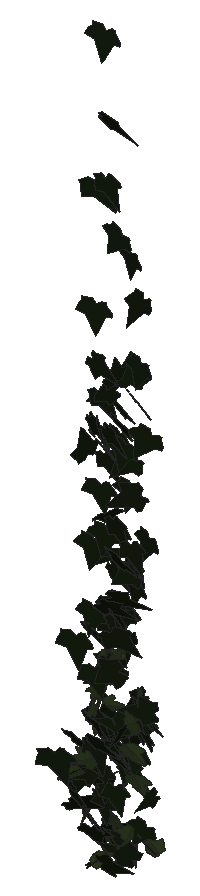
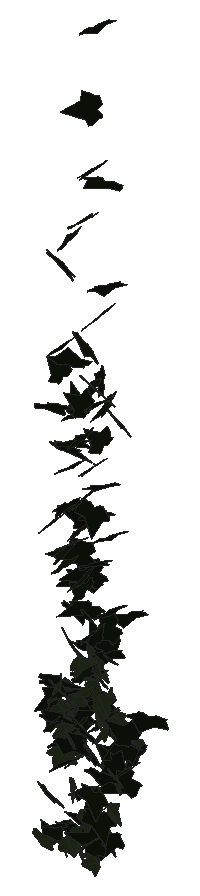
# SketchUp Ruby script. Lengths in inches.
U = 1.inch
M = Sketchup.active_model
def pt(a) = Geom::Point3d.new(a.map { |v| v * U })
def face(e, loops, mat)
  f = e.add_face(loops[0].map { |a| pt(a) })
  loops[1..].each { |l| e.add_face(l.map { |a| pt(a) }).erase! }
  f.material = f.back_material = mat if mat
  f
end
# faces: each face lists its corners as indices into pts; further lists are holes
def faces(e, pts, list, mat = nil) = list.each { |f| face(e, (f[0].is_a?(Array) ? f : [f]).map { |l| l.map { |i| pts[i] } }, mat) }
# xy, xz, yz: faces in a plane at the given z, y or x. An outline is a flat list of corners, or four numbers for a rectangle; further outlines are holes
def ring(l) = l.size == 4 ? [[l[0], l[1]], [l[2], l[1]], [l[2], l[3]], [l[0], l[3]]] : l.each_slice(2).to_a
def flat(e, list, mat, &to3) = list.each { |f| face(e, (f[0].is_a?(Array) ? f : [f]).map { |l| ring(l).map { |u, v| to3.(u, v) } }, mat) }
def xy(e, z, list, mat = nil) = flat(e, list, mat) { |x, y| [x, y, z] }
def xz(e, y, list, mat = nil) = flat(e, list, mat) { |x, z| [x, y, z] }
def yz(e, x, list, mat = nil) = flat(e, list, mat) { |y, z| [x, y, z] }
def lines(e, pts, list) = list.each { |a, b| e.add_line(pt(pts[a]), pt(pts[b])) }
# prism: a flat outline (further loops are holes) pulled along v
def prism(e, loops, v, mat = nil)
  f = face(e, loops, mat); d = Geom::Vector3d.new(v.map { |x| x * U })
  f.pushpull(f.normal.samedirection?(d) ? d.length : -d.length)
end
def box(e, o, s, mat = nil) = prism(e, [[o, [o[0] + s[0], o[1], o[2]], [o[0] + s[0], o[1] + s[1], o[2]], [o[0], o[1] + s[1], o[2]]]], [0, 0, s[2]], mat)
def at(x, y, z, deg = 0) = Geom::Transformation.translation(pt([x, y, z])) * Geom::Transformation.rotation(ORIGIN, Z_AXIS, deg.degrees)
def axes(o, x, y, z) = Geom::Transformation.new([*x, 0, *y, 0, *z, 0, *pt(o).to_a, 1])
def part(name) = M.definitions.add(name)
# library, detail: a bought-in or finely detailed component or shape, given as its bounding box
def library(name, o, s) = part(name).tap { |d| box(d.entities, o, s) }
def detail(e, o, s) = box(e.add_group.entities, o, s)
def put(e, d, t, mat = nil) = e.add_instance(d, t).tap { |i| i.material = mat if mat }
def group(e, t, mat = nil) = e.add_group.tap { |g| g.transformation = t; g.material = mat if mat }.entities
root = M.entities
M.materials.add("1026 AP 7946 SUNNY SIDE UP").color = [254, 231, 186]
M.materials.add("efeu1").color = [18, 25, 13]
M.materials.add("efeu2").color = [43, 57, 29]
c1 = part("ivyleaf_9")
p = [[1.54,2.16,1.25],[1.36,2.04,1.19],[-0.21,0.99,0.68],[-0.71,1.11,0.82],[-0.85,0.86,0.67],[-0.8,0.17,0.21],
  [-0.9,-0.01,0.1],[-0.67,-0.16,-0.02],[-0.08,-0.08,-0.05],[-0.03,-0.6,-0.4],[0.65,-0.88,-0.66],[0.83,-0.6,-0.49],
  [1.29,-0.42,-0.43],[1.8125,-0.07,-0.26],[1.21,0.44,0.15]]
faces(c1.entities,p,[[0,1,2,3,4,5,6,7,8,9,10,11,12,13,14]],"efeu1")
c2 = part("ivyleaf_10")
p = [[0,0.5,-0.03],[-0.0625,2.02,-0.43],[-0.19,2.01,-0.46],[-0.54,1.05,-0.29],[-0.52,0.625,-0.18],[-0.83,0.76,-0.28],
  [-1.16,0.64,-0.33],[-1.15,0.33,-0.24],[-0.77,-0.39,0.02],[-0.3,-0.51,0.16],[0.04,-0.48,0.23],[-0.02,2.01,-0.4375],
  [-0.06,2.01,-0.43],[0.04,-0.49,0.23],[0.67,-0.49,0.14],[1.38,0.36,-0.2],[1.375,0.51,-0.24],[0.81,0.65,-0.19],
  [0.62,0.59,-0.15],[0.6,1.09,-0.28],[0.5,1.23,-0.31]]
faces(c2.entities,p,[[0,1,2,3,4,5,6,7,8,9,10],[11,12,0,13,14,15,16,17,18,19,20]],"efeu2")
put(root,c1,axes([145.4,211.73,293.24],[0.1308,0.39329,-0.08465],[-0.1128,-0.0703,-0.41072],[-0.62235,0.0954,0.05665]),"1026 AP 7946 SUNNY SIDE UP")
put(root,c1,axes([145.09,212.38,332.73],[-0.18968,-0.4622,0.05841],[-0.00333,-0.06074,-0.49227],[0.73272,-0.11993,0.01288]),"1026 AP 7946 SUNNY SIDE UP")
put(root,c1,axes([145.11,210.46,294.86],[-0.13222,-0.37976,0.22466],[-0.00281,-0.22394,-0.39982],[0.69028,-0.07365,0.04141]),"1026 AP 7946 SUNNY SIDE UP")
put(root,c1,axes([144.88,211.98,324.96],[-0.12009,-0.34192,-0.3066],[0.40064,0.21513,-0.32283],[0.58711,-0.21674,0.15758]),"1026 AP 7946 SUNNY SIDE UP")
put(root,c2,axes([145.25,211.95,298.35],[0.15557,-0.32161,0.2261],[0.14455,-0.20269,-0.34697],[0.59659,0.13298,0.02511]),"1026 AP 7946 SUNNY SIDE UP")
put(root,c2,axes([145.39,211.61,298.87],[-0.15556,-0.36875,0.11832],[0.00302,-0.12118,-0.39266],[0.60828,-0.0937,0.03221]),"1026 AP 7946 SUNNY SIDE UP")
put(root,c1,axes([145.07,212.01,313.98],[0.16538,-0.40483,-0.15305],[0.02148,0.15363,-0.42704],[0.67649,0.09409,0.05097]),"1026 AP 7946 SUNNY SIDE UP")
put(root,c1,axes([144.89,210.25,296.61],[0.18386,-0.18869,0.33919],[0.40692,-0.21384,-0.22146],[0.43844,0.2776,0.0633]),"1026 AP 7946 SUNNY SIDE UP")
put(root,c2,axes([145.41,210.74,294.76],[0.45615,-0.26317,-0.04835],[-0.06624,0.02115,-0.40318],[0.41467,0.29287,-0.01122]),"1026 AP 7946 SUNNY SIDE UP")
put(root,c1,axes([145.48,212.25,305.9],[-0.40948,-0.27532,0.17153],[-0.06851,-0.184,-0.38115],[0.50255,-0.24941,0.08781]),"1026 AP 7946 SUNNY SIDE UP")
put(root,c1,axes([145.36,211.19,303.09],[-0.1702,-0.41187,0.10357],[-0.02747,-0.10175,-0.43922],[0.66695,-0.1093,0.00834]),"1026 AP 7946 SUNNY SIDE UP")
put(root,c1,axes([145.66,211.73,294.24],[0.0959,0.40449,0.06801],[-0.05457,0.0693,-0.41855],[-0.64155,0.05457,0.04577]),"1026 AP 7946 SUNNY SIDE UP")
put(root,c1,axes([145.59,211.95,300.43],[-0.51018,0.06694,-0.20722],[0.27988,-0.11498,-0.33523],[-0.1821,-0.36424,0.06532]),"1026 AP 7946 SUNNY SIDE UP")
put(root,c2,axes([145.53,210.68,292.96],[0.1252,-0.3432,0.1834],[0.03262,-0.1797,-0.36352],[0.60848,0.08025,-0.01825]),"1026 AP 7946 SUNNY SIDE UP")
put(root,c1,axes([145.24,212.11,302.15],[0.01326,-0.15045,0.38291],[0.13284,-0.36363,-0.15538],[0.61764,0.08144,0.0252]),"1026 AP 7946 SUNNY SIDE UP")
put(root,c1,axes([145.28,208.47,296.72],[-0.28793,-0.29848,-0.31991],[0.28394,0.25112,-0.35886],[0.61277,-0.25661,0.01597]),"1026 AP 7946 SUNNY SIDE UP")
put(root,c2,axes([145.47,211.23,297.21],[0.07716,-0.18653,-0.33902],[0.17216,0.32359,-0.1708],[0.56782,-0.07277,0.09785]),"1026 AP 7946 SUNNY SIDE UP")
put(root,c1,axes([145.94,209.99,312.04],[-0.55606,0.1642,-0.2813],[-0.36796,0.14504,0.40155],[0.34186,0.42319,-0.02534]),"1026 AP 7946 SUNNY SIDE UP")
put(root,c1,axes([145.52,210.85,291.88],[0.53458,0.1874,-0.12745],[-0.14661,-0.08851,-0.39917],[-0.32223,0.35117,-0.02983]),"1026 AP 7946 SUNNY SIDE UP")
put(root,c1,axes([145.43,209.77,302.31],[-0.19687,-0.44602,-0.09483],[0.06061,0.08211,-0.47653],[0.71274,-0.13018,0.01433]),"1026 AP 7946 SUNNY SIDE UP")
put(root,c1,axes([145.23,210.91,302.28],[0.6684,-0.16731,0.0066],[-0.01286,-0.04079,-0.46896],[0.26302,0.42318,-0.03971]),"1026 AP 7946 SUNNY SIDE UP")
put(root,c1,axes([145.48,211.08,306.72],[-0.22883,-0.42799,0.09691],[0.04251,-0.11023,-0.46226],[0.68855,-0.13543,0.06075]),"1026 AP 7946 SUNNY SIDE UP")
put(root,c1,axes([145.33,212.07,310.74],[0.2031,-0.39692,-0.07272],[0.00769,0.07331,-0.42868],[0.63325,0.12641,0.02853]),"1026 AP 7946 SUNNY SIDE UP")
put(root,c1,axes([145.26,209.25,295.16],[0.28788,-0.38308,0.20038],[0.115,-0.18295,-0.4383],[0.66727,0.1968,-0.01091]),"1026 AP 7946 SUNNY SIDE UP")
put(root,c1,axes([145.375,211.17,297.76],[0.30067,-0.38391,-0.08821],[-0.03819,0.08108,-0.44113],[0.61657,0.19224,0.01569]),"1026 AP 7946 SUNNY SIDE UP")
put(root,c1,axes([145.77,212.08,300],[-0.42041,-0.21348,0.20522],[-0.06404,-0.24165,-0.32255],[0.45595,-0.23078,0.14392]),"1026 AP 7946 SUNNY SIDE UP")
put(root,c1,axes([145.63,212.07,296.44],[-0.42852,0.00274,-0.2749],[0.41272,-0.06625,-0.27722],[-0.07591,-0.37563,0.04462]),"1026 AP 7946 SUNNY SIDE UP")
put(root,c1,axes([145.47,211.54,309.49],[-0.17974,-0.40186,-0.05058],[0.16311,0.01791,-0.41921],[0.6149,-0.12222,0.09642]),"1026 AP 7946 SUNNY SIDE UP")
put(root,c2,axes([145.43,212.05,291.04],[-0.32019,0.13339,-0.28193],[0.32063,-0.18594,-0.25008],[-0.35692,-0.28671,0.02827]),"1026 AP 7946 SUNNY SIDE UP")
put(root,c2,axes([146.01,209.11,295.79],[-0.268,-0.16531,0.31513],[-0.31549,-0.23274,-0.24536],[0.44811,-0.26273,0.01572]),"1026 AP 7946 SUNNY SIDE UP")
put(root,c1,axes([145.5625,211.1,319.15],[-0.2273,-0.4294,-0.04684],[0.0609,0.03228,-0.46578],[0.67583,-0.14732,0.02622]),"1026 AP 7946 SUNNY SIDE UP")
put(root,c1,axes([145.28,211.66,311.65],[0.18043,-0.28624,0.32071],[0.25963,-0.26845,-0.31691],[0.61424,0.19755,0.03975]),"1026 AP 7946 SUNNY SIDE UP")
put(root,c1,axes([146.11,211.74,314.55],[-0.59694,0.20463,0.01218],[-0.04521,-0.03096,-0.44247],[-0.31901,-0.37852,0.0399]),"1026 AP 7946 SUNNY SIDE UP")
put(root,c2,axes([145.68,210.69,298.47],[-0.01509,0.18356,-0.36487],[-0.01803,-0.35531,-0.19091],[-0.62846,0.00579,0.01424]),"1026 AP 7946 SUNNY SIDE UP")
put(root,c1,axes([145.52,211.89,302.38],[0.17239,-0.39335,-0.11439],[-0.05308,0.10354,-0.42004],[0.63953,0.11462,-0.00402]),"1026 AP 7946 SUNNY SIDE UP")
put(root,c2,axes([145.81,211.88,301.28],[0.189,-0.37946,-0.0446],[-0.01724,0.03968,-0.40983],[0.59992,0.12068,0.00227]),"1026 AP 7946 SUNNY SIDE UP")
put(root,c1,axes([145.53,210.83,313.25],[0.43819,-0.3393,-0.1565],[-0.18412,0.09756,-0.4509],[0.5535,0.30107,-0.02609]),"1026 AP 7946 SUNNY SIDE UP")
put(root,c1,axes([145.87,211.48,308.18],[0.18559,0.40275,-0.01505],[0.0127,-0.01997,-0.43225],[-0.63371,0.11755,-0.01307]),"1026 AP 7946 SUNNY SIDE UP")
put(root,c2,axes([146.17,210.93,300.2],[-0.30728,0.12904,0.33727],[-0.50995,0.0772,-0.23084],[-0.21199,-0.37274,0.06642]),"1026 AP 7946 SUNNY SIDE UP")
put(root,c1,axes([145.53,211.9,325.35],[0.13081,-0.44557,-0.0839],[0.00104,0.08035,-0.46622],[0.71151,0.0818,0.01611]),"1026 AP 7946 SUNNY SIDE UP")
put(root,c1,axes([145.66,211.54,293.1875],[-0.01039,-0.4155,0.06784],[0.00443,-0.06826,-0.42849],[0.66207,-0.00606,0.00393]),"1026 AP 7946 SUNNY SIDE UP")
put(root,c1,axes([145.68,209.13,295.44],[0.38112,0.25895,0.32085],[0.28705,0.25225,-0.36266],[-0.56654,0.302,0.03209]),"1026 AP 7946 SUNNY SIDE UP")
put(root,c1,axes([145.81,211.14,294.9375],[-0.43462,-0.18419,-0.20121],[0.29365,0.06741,-0.33917],[0.3016,-0.33105,0.04027]),"1026 AP 7946 SUNNY SIDE UP")
put(root,c1,axes([145.6,209.36,293.93],[0.50397,0.25496,0.25675],[0.31491,0.14616,-0.42097],[-0.4619,0.37783,-0.00687]),"1026 AP 7946 SUNNY SIDE UP")
put(root,c1,axes([145.37,212.04,328.4],[0.64545,-0.17249,0.17587],[0.22296,-0.10411,-0.45761],[0.31102,0.4326,-0.03693]),"1026 AP 7946 SUNNY SIDE UP")
put(root,c2,axes([145.77,211.98,300.59],[-0.53482,-0.1193,-0.14946],[0.27223,-0.086,-0.34742],[0.1124,-0.35936,0.1303]),"1026 AP 7946 SUNNY SIDE UP")
put(root,c1,axes([145.52,210.43,294.95],[0.0775,-0.14359,0.43338],[0.34457,-0.36134,-0.15532],[0.6095,0.22253,0.0327]),"1026 AP 7946 SUNNY SIDE UP")
put(root,c1,axes([145.68,212.38,300.34],[-0.00973,-0.28146,0.28772],[0.18315,-0.26988,-0.27753],[0.59782,0.0781,0.08971]),"1026 AP 7946 SUNNY SIDE UP")
put(root,c1,axes([146.25,210.93,291.22],[0.02533,0.02127,-0.37175],[-0.5288,0.13366,-0.00657],[0.20893,0.3357,0.02845]),"1026 AP 7946 SUNNY SIDE UP")
put(root,c1,axes([145.99,211.38,294.03],[0.18726,-0.1966,-0.37698],[-0.37293,0.27893,-0.23299],[0.53435,0.26357,-0.0305]),"1026 AP 7946 SUNNY SIDE UP")
put(root,c1,axes([145.71,211.33,291.61],[0.18689,0.33229,-0.2399],[0.05319,0.23565,0.36265],[0.63751,-0.11707,0.04007]),"1026 AP 7946 SUNNY SIDE UP")
put(root,c1,axes([145.8,212.04,305.14],[0.37061,-0.30754,-0.16514],[-0.12408,0.13901,-0.39781],[0.52973,0.24772,0.02236]),"1026 AP 7946 SUNNY SIDE UP")
put(root,c1,axes([145.93,211.78,291.68],[0.05895,-0.39281,0.03123],[-0.0112,-0.03337,-0.40657],[0.61968,0.03677,-0.01032]),"1026 AP 7946 SUNNY SIDE UP")
put(root,c1,axes([145.78,211.9,303.54],[0.10656,-0.18606,-0.4052],[0.2259,0.38426,-0.15995],[0.64421,-0.10397,0.12311]),"1026 AP 7946 SUNNY SIDE UP")
put(root,c1,axes([146.11,211.75,300.13],[-0.23541,-0.22303,0.30846],[-0.02951,-0.31896,-0.25522],[0.58792,-0.10531,0.1107]),"1026 AP 7946 SUNNY SIDE UP")
put(root,c1,axes([145.92,212.37,311.92],[0.02126,-0.38333,0.20397],[0.05638,-0.19858,-0.39544],[0.67764,0.02855,0.0265]),"1026 AP 7946 SUNNY SIDE UP")
put(root,c1,axes([146,210.45,300.48],[-0.15253,-0.37922,-0.17789],[0.08303,0.16245,-0.40217],[0.64851,-0.11,0.00965]),"1026 AP 7946 SUNNY SIDE UP")
put(root,c1,axes([146.34,211.43,299.73],[-0.52024,-0.15728,0.2068],[0.2547,0.12624,0.37599],[-0.31114,0.36631,-0.03799]),"1026 AP 7946 SUNNY SIDE UP")
put(root,c1,axes([146.6,209.41,295.91],[-0.63242,0.05212,0.11565],[-0.18362,-0.03636,-0.41493],[-0.06319,-0.41591,0.04828]),"1026 AP 7946 SUNNY SIDE UP")
put(root,c2,axes([146.18,212.1,300.73],[-0.17412,-0.36506,-0.07141],[0.11549,0.04724,-0.38851],[0.57213,-0.12064,0.05669]),"1026 AP 7946 SUNNY SIDE UP")
put(root,c1,axes([145.96,211.92,291.69],[0.0322,-0.40453,-0.0049],[0.06453,0.00452,-0.41508],[0.63281,0.02012,0.04258]),"1026 AP 7946 SUNNY SIDE UP")
put(root,c1,axes([146.16,212.18,322.52],[-0.27644,-0.31495,0.29124],[-0.0408,-0.29938,-0.35971],[0.66611,-0.14904,0.09883]),"1026 AP 7946 SUNNY SIDE UP")
put(root,c1,axes([145.75,212.26,313.55],[0.25219,-0.24995,0.33855],[0.2689,-0.28235,-0.30755],[0.59287,0.23438,-0.00452]),"1026 AP 7946 SUNNY SIDE UP")
put(root,c2,axes([146.64,209.22,296.63],[-0.34999,-0.00463,0.33],[-0.47793,-0.12028,-0.22006],[0.15929,-0.37108,0.06481]),"1026 AP 7946 SUNNY SIDE UP")
put(root,c1,axes([146.22,211.08,307.57],[-0.30368,-0.37008,-0.009],[0.03388,-0.00377,-0.42953],[0.58102,-0.19321,0.02034]),"1026 AP 7946 SUNNY SIDE UP")
put(root,c1,axes([146.1,212.125,307.28],[0.07597,-0.40901,0.12389],[0.01978,-0.12194,-0.425],[0.6711,0.04989,-0.0015]),"1026 AP 7946 SUNNY SIDE UP")
put(root,c2,axes([146.53,211.22,292.64],[-0.48675,0.19775,0.09001],[-0.15265,0.00703,-0.37551],[-0.30294,-0.32127,0.0446]),"1026 AP 7946 SUNNY SIDE UP")
put(root,c1,axes([146.36,211.53,296.86],[-0.42125,0.2828,0.18151],[0.21295,-0.11188,0.40015],[0.47722,0.29955,-0.01834]),"1026 AP 7946 SUNNY SIDE UP")
put(root,c1,axes([146.83,212.1,296.7],[-0.07035,0.12268,-0.37154],[-0.29523,-0.32382,-0.0912],[-0.52239,0.16648,0.10158]),"1026 AP 7946 SUNNY SIDE UP")
put(root,c1,axes([146.86,210.95,315.82],[-0.48085,0.17834,-0.32537],[-0.38099,0.20873,0.36317],[0.42626,0.38774,-0.04245]),"1026 AP 7946 SUNNY SIDE UP")
put(root,c1,axes([146.81,209.69,291.19],[-0.17304,0.36837,0.00013],[-0.02155,-0.00615,-0.39581],[-0.57884,-0.10989,0.0147]),"1026 AP 7946 SUNNY SIDE UP")
put(root,c1,axes([146.43,211.375,294.01],[-0.09709,-0.37121,-0.12306],[0.06119,0.11233,-0.38651],[0.60909,-0.07046,0.01921]),"1026 AP 7946 SUNNY SIDE UP")
put(root,c1,axes([146.58,211.02,298.4],[-0.19186,-0.09951,0.44541],[-0.13185,-0.43573,-0.13007],[0.68592,-0.11159,0.09959]),"1026 AP 7946 SUNNY SIDE UP")
put(root,c1,axes([146.97,211.23,300.57],[-0.52339,0.20405,-0.00247],[-0.02187,-0.02946,-0.401],[-0.32014,-0.33157,0.03142]),"1026 AP 7946 SUNNY SIDE UP")
put(root,c1,axes([146.25,208.75,294.81],[0.32621,-0.37272,0.15984],[0.09945,-0.14469,-0.44005],[0.62828,0.21642,-0.01334]),"1026 AP 7946 SUNNY SIDE UP")
put(root,c2,axes([146.72,211.94,294.49],[0.15685,-0.31105,-0.20951],[-0.04294,0.20204,-0.33387],[0.58125,0.09886,0.03187]),"1026 AP 7946 SUNNY SIDE UP")
put(root,c1,axes([146.68,211.87,303.16],[-0.54754,-0.07765,-0.19756],[0.30397,0.00923,-0.36626],[0.11411,-0.39721,0.0277]),"1026 AP 7946 SUNNY SIDE UP")
put(root,c2,axes([146.49,210.67,298.75],[-0.09864,-0.10888,-0.39494],[0.34494,0.31381,-0.12717],[0.52203,-0.22793,0.0094]),"1026 AP 7946 SUNNY SIDE UP")
put(root,c1,axes([146.42,209.91,317.1],[0.40131,-0.28761,-0.26896],[-0.14506,0.25662,-0.38506],[0.59152,0.25806,0.08804]),"1026 AP 7946 SUNNY SIDE UP")
put(root,c2,axes([146.81,212.1,291.64],[-0.30666,-0.28547,0.13304],[-0.01588,-0.14815,-0.34958],[0.49347,-0.18217,0.07143]),"1026 AP 7946 SUNNY SIDE UP")
put(root,c1,axes([147.14,210.72,300.66],[-0.71468,0.00813,0.1115],[-0.17055,-0.04525,-0.46618],[0.0041,-0.46502,0.04456]),"1026 AP 7946 SUNNY SIDE UP")
put(root,c1,axes([146.51,209.89,297.02],[0.02895,-0.45955,-0.06584],[-0.02807,0.0606,-0.47319],[0.72845,0.0206,-0.01562]),"1026 AP 7946 SUNNY SIDE UP")
put(root,c2,axes([146.69,212.23,296.96],[0.40403,-0.26976,0.08557],[0.06355,-0.07809,-0.38346],[0.43997,0.259,-0.02319]),"1026 AP 7946 SUNNY SIDE UP")
put(root,c2,axes([146.53,210.08,291.01],[0.24999,0.21737,0.28113],[0.2005,0.24148,-0.27453],[-0.509,0.20188,0.02993]),"1026 AP 7946 SUNNY SIDE UP")
put(root,c1,axes([146.57,212.39,321.59],[0.01868,-0.38663,0.25678],[-0.00681,-0.25161,-0.39982],[0.72516,0.0076,-0.01037]),"1026 AP 7946 SUNNY SIDE UP")
put(root,c2,axes([146.7,211.47,291.03],[0.29251,-0.27869,0.17732],[0.14609,-0.14682,-0.34602],[0.49526,0.20791,-0.00266]),"1026 AP 7946 SUNNY SIDE UP")
put(root,c1,axes([146.95,211.93,315.23],[-0.63533,-0.06591,0.20629],[0.30314,0.06162,0.42121],[-0.1355,0.44689,-0.02493]),"1026 AP 7946 SUNNY SIDE UP")
put(root,c2,axes([146.86,211.48,296.16],[-0.04181,-0.1387,-0.37281],[0.1158,0.35351,-0.14341],[0.59711,-0.07827,0.00171]),"1026 AP 7946 SUNNY SIDE UP")
put(root,c1,axes([147.03,211.9,311.22],[-0.50101,-0.26302,0.15484],[-0.10262,-0.15558,-0.41973],[0.46635,-0.3168,0.07399]),"1026 AP 7946 SUNNY SIDE UP")
put(root,c1,axes([146.5,210.11,313.66],[0.10692,-0.06608,-0.45717],[0.64661,-0.16938,0.08998],[-0.28068,-0.41538,0.03314]),"1026 AP 7946 SUNNY SIDE UP")
put(root,c1,axes([146.74,212.15,301.72],[-0.33743,-0.03414,-0.35369],[0.52529,-0.12074,-0.20357],[-0.13436,-0.38628,0.09239]),"1026 AP 7946 SUNNY SIDE UP")
put(root,c1,axes([146.6,211.63,312.86],[-0.15027,-0.10409,0.42025],[0.25831,-0.39497,-0.0664],[0.61049,0.1415,0.13153]),"1026 AP 7946 SUNNY SIDE UP")
put(root,c1,axes([146.53,211.4,296.1875],[-0.11794,-0.10421,-0.37802],[0.58944,0.04587,-0.09224],[0.10597,-0.37112,0.09236]),"1026 AP 7946 SUNNY SIDE UP")
put(root,c1,axes([146.625,211.52,297.16],[0.27109,-0.36826,-0.032],[-0.03739,0.02084,-0.41858],[0.57965,0.17357,-0.01203]),"1026 AP 7946 SUNNY SIDE UP")
put(root,c1,axes([146.625,211.55,296.08],[0.14969,-0.29986,0.23399],[0.09252,-0.22132,-0.32528],[0.58586,0.11157,-0.00841]),"1026 AP 7946 SUNNY SIDE UP")
put(root,c1,axes([146.78,211.63,295.47],[-0.01272,-0.36006,0.17722],[-0.01155,-0.17394,-0.37203],[0.62874,-0.01048,-0.00325]),"1026 AP 7946 SUNNY SIDE UP")
put(root,c1,axes([146.51,209.54,297.39],[0.53824,-0.06406,0.17847],[0.25351,-0.07594,-0.3568],[0.14281,0.37623,-0.03928]),"1026 AP 7946 SUNNY SIDE UP")
put(root,c1,axes([146.72,211,308.22],[0.26936,-0.42693,-0.08581],[-0.06427,0.07071,-0.47335],[0.68022,0.17574,-0.01075]),"1026 AP 7946 SUNNY SIDE UP")
put(root,c1,axes([146.76,210.36,313.35],[0.43891,-0.33013,-0.12555],[-0.08972,0.10862,-0.44396],[0.54499,0.28375,0.02802]),"1026 AP 7946 SUNNY SIDE UP")
put(root,c1,axes([147.55,210.78,297.93],[-0.26412,-0.00715,0.35851],[-0.52765,-0.09952,-0.16953],[0.14567,-0.37343,0.03597]),"1026 AP 7946 SUNNY SIDE UP")
put(root,c1,axes([146.68,210.25,304.19],[0.59118,0.08566,0.22377],[0.34718,0.00066,-0.39486],[-0.11721,0.43396,-0.04093]),"1026 AP 7946 SUNNY SIDE UP")
put(root,c2,axes([147.57,211.95,298.125],[-0.40167,0.05348,0.29559],[-0.44538,-0.13589,-0.23475],[0.10872,-0.35908,0.13041]),"1026 AP 7946 SUNNY SIDE UP")
put(root,c2,axes([147.22,211.15,298.15],[-0.18785,-0.34202,-0.13897],[0.11084,0.11583,-0.37153],[0.56625,-0.13614,0.02662]),"1026 AP 7946 SUNNY SIDE UP")
put(root,c1,axes([146.84,210.93,303.55],[0.2259,-0.35388,0.24387],[0.13827,-0.22195,-0.39476],[0.65683,0.16844,-0.00077]),"1026 AP 7946 SUNNY SIDE UP")
put(root,c2,axes([147.27,211.13,291.36],[0.05157,-0.28777,0.27039],[0.0515,-0.26207,-0.2999],[0.612,0.0463,0.00245]),"1026 AP 7946 SUNNY SIDE UP")
put(root,c1,axes([147.17,211.21,312.29],[-0.20471,-0.40028,0.11498],[-0.02715,-0.11403,-0.43389],[0.65382,-0.13006,0.01799]),"1026 AP 7946 SUNNY SIDE UP")
put(root,c1,axes([147.15,211.68,309.875],[-0.18404,-0.39637,0.14442],[-0.01082,-0.14602,-0.42527],[0.66218,-0.11255,0.03319]),"1026 AP 7946 SUNNY SIDE UP")
put(root,c1,axes([146.99,212.06,305.84],[0.19625,-0.38486,0.09266],[0.02111,-0.09243,-0.41705],[0.62189,0.12459,-0.01508]),"1026 AP 7946 SUNNY SIDE UP")
put(root,c1,axes([147.18,212.36,316.05],[-0.10089,-0.39906,0.1728],[-0.05427,-0.16661,-0.4173],[0.67989,-0.07252,-0.00766]),"1026 AP 7946 SUNNY SIDE UP")
put(root,c1,axes([147.58,211.98,298.99],[-0.55506,0.09739,-0.12228],[0.15229,-0.09141,-0.3728],[-0.18819,-0.36121,0.05897]),"1026 AP 7946 SUNNY SIDE UP")
put(root,c1,axes([147.8,212.27,297.63],[-0.49754,-0.02477,0.22291],[-0.33407,-0.04991,-0.32604],[0.07628,-0.38014,0.02601]),"1026 AP 7946 SUNNY SIDE UP")
put(root,c1,axes([147.1875,211.96,297.73],[0.08436,-0.3815,-0.03171],[-0.02113,0.02699,-0.3966],[0.60118,0.05448,-0.00949]),"1026 AP 7946 SUNNY SIDE UP")
put(root,c1,axes([147.11,211.55,295.31],[0.18877,-0.31622,-0.19774],[0.04734,0.20769,-0.33501],[0.57825,0.08622,0.09198]),"1026 AP 7946 SUNNY SIDE UP")
put(root,c1,axes([147.93,210.68,291.18],[-0.18845,0.0841,0.39079],[-0.59223,0.07038,-0.13843],[-0.1471,-0.39108,0.05666]),"1026 AP 7946 SUNNY SIDE UP")
put(root,c1,axes([147.56,211.33,305.69],[-0.38152,-0.21274,0.29111],[-0.14733,-0.29317,-0.31066],[0.53788,-0.2312,0.12139]),"1026 AP 7946 SUNNY SIDE UP")
put(root,c1,axes([147.59,210.72,297.84],[-0.20375,0.09879,-0.35946],[0.27372,-0.30876,-0.15822],[-0.50119,-0.20879,0.05972]),"1026 AP 7946 SUNNY SIDE UP")
put(root,c1,axes([147.36,211.75,304.875],[-0.10143,-0.34162,0.22673],[0.04631,-0.22811,-0.35411],[0.63898,-0.0377,0.06165]),"1026 AP 7946 SUNNY SIDE UP")
put(root,c2,axes([147.49,211.86,299.2],[-0.08775,0.34236,-0.21218],[0.01381,-0.20881,-0.35789],[-0.62966,-0.05229,0.02172]),"1026 AP 7946 SUNNY SIDE UP")
put(root,c1,axes([147.53,211.69,296.16],[-0.21205,-0.36099,0.04618],[-0.00544,-0.04871,-0.39703],[0.57237,-0.1342,0.01334]),"1026 AP 7946 SUNNY SIDE UP")
put(root,c1,axes([147.23,208.58,294.0625],[0.17604,-0.21936,0.31248],[0.20615,-0.27495,-0.25526],[0.55301,0.17232,-0.00431]),"1026 AP 7946 SUNNY SIDE UP")
put(root,c2,axes([147.4375,211.65,291.07],[0.25069,-0.194,0.29033],[0.31251,-0.20205,-0.25929],[0.43965,0.25424,0.01877]),"1026 AP 7946 SUNNY SIDE UP")
put(root,c1,axes([147.69,212.07,292.12],[-0.35924,-0.27313,0.10663],[-0.0054,-0.13078,-0.3587],[0.46012,-0.21478,0.07905]),"1026 AP 7946 SUNNY SIDE UP")
put(root,c1,axes([147.27,210.0625,296.75],[0.51395,-0.17376,0.11054],[0.11861,-0.08743,-0.37961],[0.29928,0.33304,-0.03937]),"1026 AP 7946 SUNNY SIDE UP")
put(root,c2,axes([147.43,211.2,296.54],[-0.45382,-0.06935,-0.26121],[0.41226,-0.05802,-0.29189],[0.0199,-0.37951,0.09001]),"1026 AP 7946 SUNNY SIDE UP")
put(root,c1,axes([147.16,210.4,306.81],[0.37284,-0.23129,0.31237],[0.34159,-0.21341,-0.34248],[0.49484,0.32158,0.00106]),"1026 AP 7946 SUNNY SIDE UP")
put(root,c2,axes([148.11,210.69,298.3125],[-0.32543,0.08333,0.32674],[-0.50993,-0.00018,-0.21829],[-0.07143,-0.37832,0.06975]),"1026 AP 7946 SUNNY SIDE UP")
put(root,c1,axes([147.21,209.64,291.12],[0.24802,-0.04406,0.36149],[0.46927,-0.19006,-0.16378],[0.29908,0.33475,-0.04279]),"1026 AP 7946 SUNNY SIDE UP")
put(root,c1,axes([147.84,211.65,319.96],[-0.65969,0.03322,-0.2352],[0.35013,-0.06716,-0.43165],[-0.09605,-0.47299,0.04193]),"1026 AP 7946 SUNNY SIDE UP")
put(root,c1,axes([147.44,212,298.47],[0.22915,-0.34502,0.13074],[0.06738,-0.12176,-0.38648],[0.57518,0.15172,-0.00681]),"1026 AP 7946 SUNNY SIDE UP")
put(root,c1,axes([147.67,212.34,307.1],[-0.09393,-0.34864,0.22973],[-0.03689,-0.2241,-0.36549],[0.65139,-0.06296,0.01243]),"1026 AP 7946 SUNNY SIDE UP")
put(root,c1,axes([147.4,211.79,314.42],[0.11645,-0.2712,0.35838],[0.24891,-0.31457,-0.28792],[0.64943,0.16919,0.04609]),"1026 AP 7946 SUNNY SIDE UP")
put(root,c1,axes([147.29,210.21,304.81],[0.50515,0.04454,0.31349],[0.47986,0.00527,-0.33296],[-0.05659,0.4423,-0.02498]),"1026 AP 7946 SUNNY SIDE UP")
put(root,c1,axes([148.25,210.85,310.22],[-0.6829,0.00199,0.10857],[-0.16518,-0.04424,-0.44543],[0.01337,-0.44471,0.04217]),"1026 AP 7946 SUNNY SIDE UP")
put(root,c1,axes([148.09,212.18,293.83],[-0.50887,0.11672,-0.1342],[0.14991,-0.11359,-0.34775],[-0.23151,-0.33011,0.06981]),"1026 AP 7946 SUNNY SIDE UP")
put(root,c1,axes([147.59,212.01,297.15],[0.09216,-0.31428,0.26957],[0.13517,-0.2508,-0.3294],[0.63052,0.09971,0.03121]),"1026 AP 7946 SUNNY SIDE UP")
put(root,c1,axes([148.03,211.99,312.78],[-0.53027,-0.26822,0.01783],[0.03801,-0.06034,-0.4396],[0.42108,-0.33233,0.06214]),"1026 AP 7946 SUNNY SIDE UP")
put(root,c1,axes([147.62,208.28,299.18],[0.60666,-0.23589,-0.15551],[0.25748,-0.01569,0.46042],[-0.35585,-0.41351,0.06803]),"1026 AP 7946 SUNNY SIDE UP")
put(root,c2,axes([147.93,211.09,295.19],[-0.56875,-0.08677,-0.09248],[0.14789,-0.0107,-0.38189],[0.12827,-0.37241,0.03022]),"1026 AP 7946 SUNNY SIDE UP")
put(root,c2,axes([148.34,212.06,291.2],[0.30665,0.07085,0.32676],[-0.50851,0.01055,0.20273],[0.044,-0.37185,0.06575]),"1026 AP 7946 SUNNY SIDE UP")
put(root,c1,axes([147.66,211.64,298.21],[0.60517,-0.07001,0.03217],[0.03779,-0.04374,-0.40129],[0.11474,0.38368,-0.03753]),"1026 AP 7946 SUNNY SIDE UP")
put(root,c1,axes([148.54,211.41,298.71],[-0.45229,0.00124,0.30239],[-0.45853,-0.04809,-0.29447],[0.05265,-0.40815,0.03319]),"1026 AP 7946 SUNNY SIDE UP")
put(root,c1,axes([147.86,210.8125,307.43],[0.05584,-0.39604,-0.13968],[-0.02293,0.13257,-0.40885],[0.65668,0.03831,-0.0024]),"1026 AP 7946 SUNNY SIDE UP")
put(root,c1,axes([147.73,211.96,291.32],[0.0177,-0.19061,0.34229],[0.26434,-0.29738,-0.18277],[0.54285,0.15102,0.07784]),"1026 AP 7946 SUNNY SIDE UP")
put(root,c1,axes([147.71,209.66,303.31],[-0.00313,-0.15085,-0.41497],[0.35706,0.34076,-0.13092],[0.57291,-0.2132,0.07932]),"1026 AP 7946 SUNNY SIDE UP")
